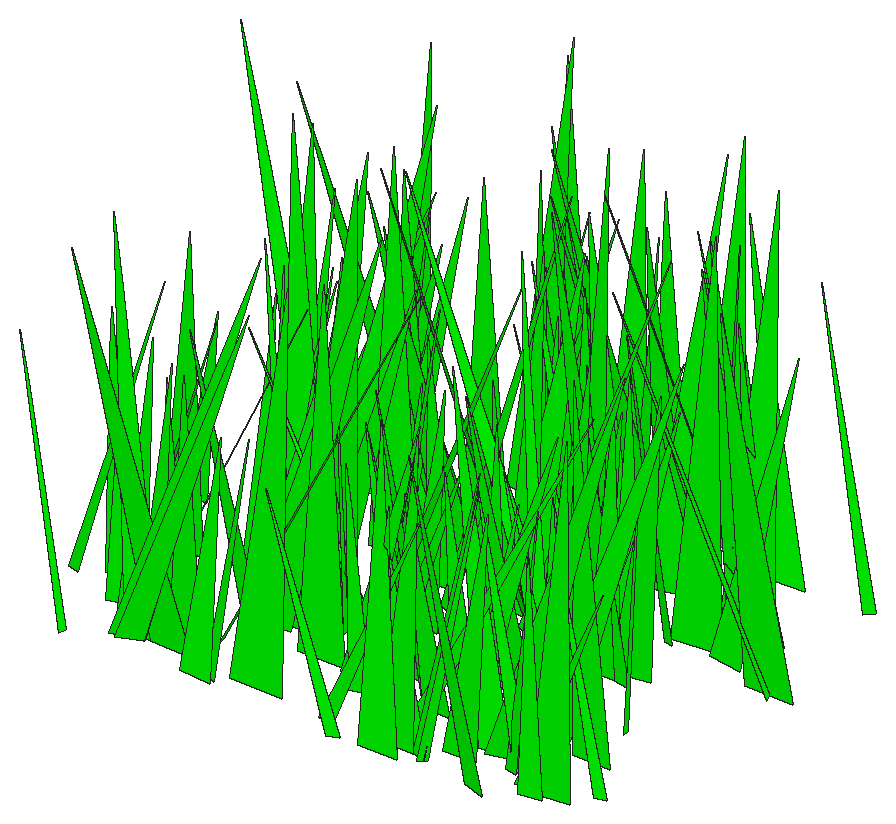
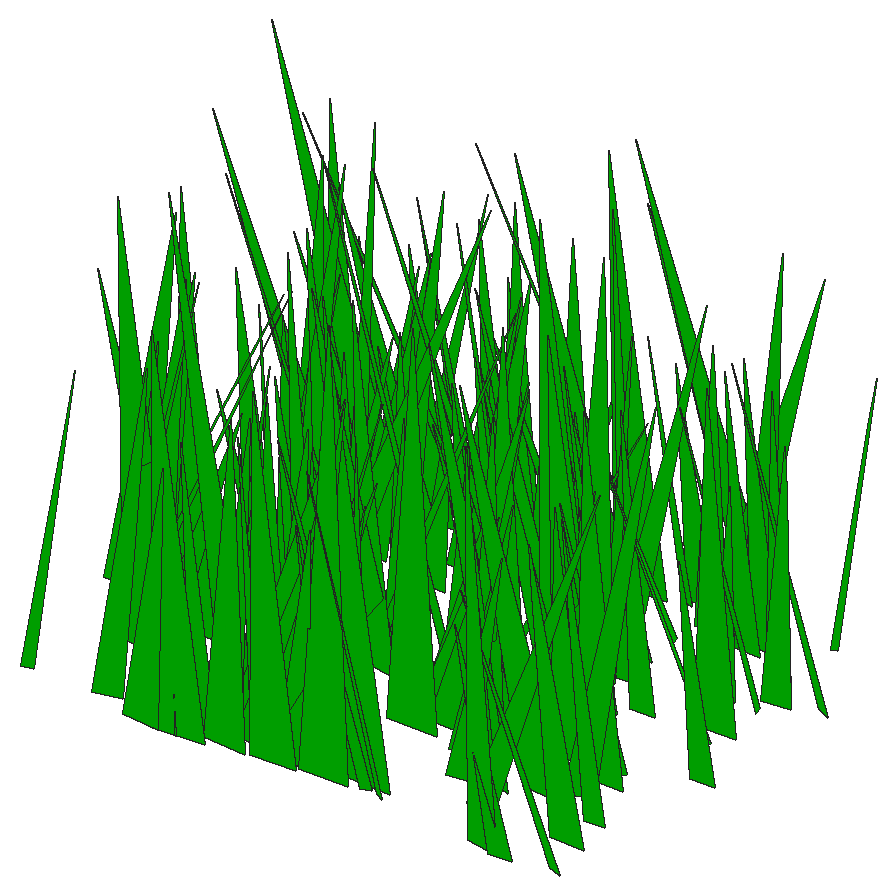
# SketchUp Ruby script. Lengths in inches.
U = 1.inch
M = Sketchup.active_model
def pt(a) = Geom::Point3d.new(a.map { |v| v * U })
def face(e, loops, mat)
  f = e.add_face(loops[0].map { |a| pt(a) })
  loops[1..].each { |l| e.add_face(l.map { |a| pt(a) }).erase! }
  f.material = f.back_material = mat if mat
  f
end
# faces: each face lists its corners as indices into pts; further lists are holes
def faces(e, pts, list, mat = nil) = list.each { |f| face(e, (f[0].is_a?(Array) ? f : [f]).map { |l| l.map { |i| pts[i] } }, mat) }
# xy, xz, yz: faces in a plane at the given z, y or x. An outline is a flat list of corners, or four numbers for a rectangle; further outlines are holes
def ring(l) = l.size == 4 ? [[l[0], l[1]], [l[2], l[1]], [l[2], l[3]], [l[0], l[3]]] : l.each_slice(2).to_a
def flat(e, list, mat, &to3) = list.each { |f| face(e, (f[0].is_a?(Array) ? f : [f]).map { |l| ring(l).map { |u, v| to3.(u, v) } }, mat) }
def xy(e, z, list, mat = nil) = flat(e, list, mat) { |x, y| [x, y, z] }
def xz(e, y, list, mat = nil) = flat(e, list, mat) { |x, z| [x, y, z] }
def yz(e, x, list, mat = nil) = flat(e, list, mat) { |y, z| [x, y, z] }
def lines(e, pts, list) = list.each { |a, b| e.add_line(pt(pts[a]), pt(pts[b])) }
# prism: a flat outline (further loops are holes) pulled along v
def prism(e, loops, v, mat = nil)
  f = face(e, loops, mat); d = Geom::Vector3d.new(v.map { |x| x * U })
  f.pushpull(f.normal.samedirection?(d) ? d.length : -d.length)
end
def box(e, o, s, mat = nil) = prism(e, [[o, [o[0] + s[0], o[1], o[2]], [o[0] + s[0], o[1] + s[1], o[2]], [o[0], o[1] + s[1], o[2]]]], [0, 0, s[2]], mat)
def at(x, y, z, deg = 0) = Geom::Transformation.translation(pt([x, y, z])) * Geom::Transformation.rotation(ORIGIN, Z_AXIS, deg.degrees)
def axes(o, x, y, z) = Geom::Transformation.new([*x, 0, *y, 0, *z, 0, *pt(o).to_a, 1])
def part(name) = M.definitions.add(name)
# library, detail: a bought-in or finely detailed component or shape, given as its bounding box
def library(name, o, s) = part(name).tap { |d| box(d.entities, o, s) }
def detail(e, o, s) = box(e.add_group.entities, o, s)
def put(e, d, t, mat = nil) = e.add_instance(d, t).tap { |i| i.material = mat if mat }
def group(e, t, mat = nil) = e.add_group.tap { |g| g.transformation = t; g.material = mat if mat }.entities
root = M.entities
M.materials.add("[0065_Lime]").color = [0, 255, 0]
c1 = part("fur_instance\#9")
p = [[0.8125,0,1.79],[0.67,-0.02,1.48],[0,-0.11,0],[0,0.11,0]]
faces(c1.entities,p,[[0,1,2,3]])
put(root,c1,axes([28.53,26.51,1.48],[1.94446,-0.52431,0.30164],[3.73909,0.27553,0.10032],[-0.2811,0.03815,3.42098]),"[0065_Lime]")
put(root,c1,axes([30.69,29.18,1.48],[-7.24883,0.59659,1.35662],[-4.26048,-1.0427,0.30299],[1.62965,-0.07228,6.8265]),"[0065_Lime]")
put(root,c1,axes([29.66,21.89,1.48],[2.43602,-0.54167,1.98048],[4.36192,0.38979,0.02249],[-1.32716,0.28686,3.70911]),"[0065_Lime]")
put(root,c1,axes([30.3125,18.52,1.48],[-5.37526,0.04391,1.37175],[-0.43696,-0.7889,-0.28668],[1.65853,-0.06553,4.3703]),"[0065_Lime]")
put(root,c1,axes([29.3,31.42,1.48],[1.7372,0.77211,0.89596],[-5.60051,0.24495,0.11135],[-0.19907,-0.15344,4.68622]),"[0065_Lime]")
put(root,c1,axes([28.375,21.41,1.48],[6.02853,0.28698,0.82516],[-2.03066,0.85892,-0.1937],[-1.03751,-0.01361,5.17381]),"[0065_Lime]")
put(root,c1,axes([29.4,30.12,1.48],[4.78763,-0.38115,1.16224],[2.70623,0.70036,0.32035],[-1.44058,0.04897,4.46442]),"[0065_Lime]")
put(root,c1,axes([28.59,32.84,1.48],[4.66829,0.30685,0.32277],[-2.18537,0.65817,-0.05356],[-0.38739,-0.01522,4.19181]),"[0065_Lime]")
put(root,c1,axes([30.03,24.08,1.48],[0.66516,-0.9095,1.03335],[6.5959,0.0908,-0.13111],[0.03354,0.17988,5.29092]),"[0065_Lime]")
put(root,c1,axes([32.3,31.47,1.48],[-5.59806,-0.65347,0.48872],[4.67301,-0.78835,0.09346],[0.38843,0.0664,5.91905]),"[0065_Lime]")
put(root,c1,axes([30.49,20.73,1.48],[-3.94514,0.41383,2.08396],[-3.38186,-0.61798,-0.12382],[1.94941,-0.23458,4.00264]),"[0065_Lime]")
put(root,c1,axes([30.72,28.24,1.48],[0.06351,1.00668,1.49718],[-7.39594,0.00488,0.09759],[0.10756,-0.25875,5.82675]),"[0065_Lime]")
put(root,c1,axes([31.03,22.45,1.48],[1.96058,-0.48802,0.89851],[3.52754,0.2984,0.33812],[-0.91568,0.10464,3.22638]),"[0065_Lime]")
put(root,c1,axes([29.83,22.45,1.48],[5.47637,0.03064,0.82466],[-0.13545,0.78027,-0.37615],[-1.02812,0.06038,4.44218]),"[0065_Lime]")
put(root,c1,axes([30.23,33.19,1.48],[2.61824,-0.49944,0.0051],[3.55197,0.36771,0.12511],[-0.12755,-0.01211,3.58864]),"[0065_Lime]")
put(root,c1,axes([30.96,33.04,1.48],[5.28712,0.68809,2.30985],[-5.25194,0.79999,-0.03173],[-2.11186,-0.26682,5.86172]),"[0065_Lime]")
put(root,c1,axes([30.54,27.5625,1.48],[4.55578,-0.22354,0.90925],[1.72318,0.64956,-0.3614],[-0.90051,0.11206,3.90849]),"[0065_Lime]")
put(root,c1,axes([32.23,19.62,1.48],[-5.92887,0.69451,1.85297],[-5.05854,-0.87786,0.31647],[2.00728,-0.16093,6.27061]),"[0065_Lime]")
put(root,c1,axes([33.25,19.58,1.48],[-3.84627,-0.95409,0.5057],[6.81766,-0.53944,0.20488],[0.08641,0.09347,6.34419]),"[0065_Lime]")
put(root,c1,axes([29.71,24.71,1.48],[5.7731,0.03624,0.21564],[-0.26747,0.81149,0.16836],[-0.25542,-0.03075,4.69758]),"[0065_Lime]")
put(root,c1,axes([31.66,19.78,1.48],[2.95946,0.67914,1.09682],[-4.91075,0.4372,-0.30431],[-1.03058,-0.13302,4.59976]),"[0065_Lime]")
put(root,c1,axes([32.21,27.77,1.48],[-0.65846,0.74084,0.40123],[-5.28493,-0.09631,0.22017],[0.33079,-0.06396,4.31622]),"[0065_Lime]")
put(root,c1,axes([32.08,20.09,1.48],[3.00252,0.56147,1.53129],[-4.31475,0.44126,0.17608],[-0.94492,-0.23081,4.06171]),"[0065_Lime]")
put(root,c1,axes([31.38,29.75,1.48],[3.30997,1.06959,0.29263],[-7.6179,0.46583,-0.04234],[-0.19124,-0.04344,6.75146]),"[0065_Lime]")
put(root,c1,axes([32.22,24.5,1.48],[4.33729,-0.47684,1.24563],[3.42635,0.64049,0.32223],[-1.45633,0.08675,4.46792]),"[0065_Lime]")
put(root,c1,axes([33.83,30.44,1.48],[-2.98341,0.56809,0.39795],[-4.05646,-0.42208,0.06879],[0.35882,-0.04822,4.08637]),"[0065_Lime]")
put(root,c1,axes([32.56,30.17,1.48],[5.09678,0.33329,1.41012],[-2.41603,0.75303,-0.18614],[-1.67146,-0.07218,4.56892]),"[0065_Lime]")
put(root,c1,axes([33.7,24.95,1.48],[4.55404,-0.88484,3.54342],[7.25802,0.72573,-0.0992],[-2.43922,0.50746,6.32039]),"[0065_Lime]")
put(root,c1,axes([34.61,29.27,1.48],[-3.27427,0.6261,0.62858],[-4.50578,-0.46309,-0.07276],[0.38476,-0.09501,4.49706]),"[0065_Lime]")
put(root,c1,axes([34.05,23.73,1.48],[-6.2833,0.18815,2.07275],[-1.57652,-0.94423,-0.28991],[2.4085,-0.12721,5.21763]),"[0065_Lime]")
put(root,c1,axes([33.74,29.49,1.48],[1.85607,-0.86738,1.7738],[6.48186,0.28817,0.23426],[-0.91846,0.28085,5.23782]),"[0065_Lime]")
put(root,c1,axes([33.59,19.78,1.48],[-1.27012,-0.73073,1.17098],[5.35552,-0.19609,-0.25694],[0.65873,0.18526,4.34675]),"[0065_Lime]")
put(root,c1,axes([32.92,25.06,1.48],[5.95801,-0.23794,1.35455],[1.62666,0.86929,0.38291],[-1.73046,-0.0021,5.02369]),"[0065_Lime]")
put(root,c1,axes([34.58,25.33,1.48],[-3.2959,0.39537,0.88114],[-2.93786,-0.47183,-0.17664],[0.67751,-0.12263,3.52053]),"[0065_Lime]")
put(root,c1,axes([34.32,29.35,1.48],[-2.83799,-0.41183,0.81012],[2.91692,-0.41935,-0.38255],[1.03599,0.05255,3.29636]),"[0065_Lime]")
put(root,c1,axes([32,19.32,1.48],[6.93626,-0.5454,0.40087],[3.86444,0.97705,0.30254],[-0.61157,-0.01192,6.45823]),"[0065_Lime]")
put(root,c1,axes([31.9,19.36,1.48],[7.73818,-0.67451,0.62273],[4.80985,1.09173,0.07932],[-0.70212,0.04502,7.40659]),"[0065_Lime]")
put(root,c1,axes([33.5,23.36,1.48],[1.89489,0.68749,0.51615],[-4.93049,0.26052,0.34847],[0.17399,-0.10477,4.2535]),"[0065_Lime]")
put(root,c1,axes([33.64,25.6,1.48],[1.01521,-1.0318,0.08282],[7.32975,0.14149,-0.38137],[0.45056,0.02317,6.01754]),"[0065_Lime]")
put(root,c1,axes([34.68,27.48,1.48],[-0.23063,1.04261,2.1931],[-7.89444,-0.03172,-0.04394],[0.02632,-0.37892,6.03813]),"[0065_Lime]")
put(root,c1,axes([36.03,20.11,1.48],[3.99965,0.43225,3.3723],[-4.14694,0.70794,0.21354],[-3.07471,-0.39253,4.09875]),"[0065_Lime]")
put(root,c1,axes([36.26,28.41,1.48],[-3.72702,-0.90922,0.02059],[6.46597,-0.52349,-0.21624],[0.24299,-0.01556,6.07]),"[0065_Lime]")
put(root,c1,axes([34.71,18.79,1.48],[-0.08844,0.67947,0.57665],[-4.87322,-0.01979,0.2867],[0.3691,-0.09842,3.92345]),"[0065_Lime]")
put(root,c1,axes([37.39,23.35,1.48],[-5.60505,0.08473,0.07621],[-0.6068,-0.78679,-0.21423],[0.06488,-0.03821,4.58052]),"[0065_Lime]")
put(root,c1,axes([33.75,26.15,1.48],[4.79267,-0.55779,0.71821],[4.03311,0.67653,-0.20055],[-0.52063,0.10603,5.05799]),"[0065_Lime]")
put(root,c1,axes([35.7,24.08,1.48],[-0.55954,-0.6155,0.93138],[4.52001,-0.06669,0.31996],[-0.25857,0.1662,3.57759]),"[0065_Lime]")
put(root,c1,axes([34.34,25,1.48],[2.28445,-1.28329,0.05879],[9.13284,0.32099,-0.01488],[0.00021,0.01048,7.65741]),"[0065_Lime]")
put(root,c1,axes([33.98,28.3,1.48],[5.70355,-0.61239,1.36982],[4.55179,0.81253,-0.36773],[-1.05353,0.19523,5.82706]),"[0065_Lime]")
put(root,c1,axes([36.7,28.6,1.48],[-4.02898,-0.33853,0.43606],[2.44192,-0.56771,0.15975],[0.35826,0.06247,3.81507]),"[0065_Lime]")
put(root,c1,axes([35.05,19,1.48],[4.38399,0.26521,1.15978],[-2.01567,0.63966,0.13987],[-1.2378,-0.10234,3.87989]),"[0065_Lime]")
put(root,c1,axes([35.45,22.61,1.48],[-0.06957,-0.57004,1.65432],[4.524,-0.03113,-0.23356],[0.35594,0.28425,3.29199]),"[0065_Lime]")
put(root,c1,axes([35.97,32.21,1.48],[4.6183,0.51196,2.26448],[-4.10413,0.70913,0.1659],[-2.0446,-0.26704,4.78195]),"[0065_Lime]")
put(root,c1,axes([35.71,20.77,1.48],[-6.79525,0.23703,2.95559],[-2.08303,-1.06784,-0.29908],[3.42187,-0.17934,5.68724]),"[0065_Lime]")
put(root,c1,axes([34.9,32.57,1.48],[5.67197,0.20058,0.98782],[-1.44711,0.81436,-0.04321],[-1.19089,-0.03425,4.75732]),"[0065_Lime]")
put(root,c1,axes([36.37,23.27,1.48],[-4.35434,-0.01055,1.51071],[-0.07069,-0.66331,-0.29006],[1.85742,-0.04998,3.53051]),"[0065_Lime]")
put(root,c1,axes([35.56,32.3,1.48],[4.79175,1.02399,2.56946],[-7.82384,0.6978,0.33523],[-1.36735,-0.4043,7.08626]),"[0065_Lime]")
put(root,c1,axes([36.38,31.375,1.48],[2.96702,0.50866,1.34988],[-3.82227,0.44536,-0.06482],[-1.11723,-0.1728,3.80663]),"[0065_Lime]")
put(root,c1,axes([36.8125,32.4375,1.48],[-0.23189,-0.64567,0.15021],[4.59656,-0.03176,0.12023],[-0.13844,0.02695,3.74041]),"[0065_Lime]")
put(root,c1,axes([34.47,22.27,1.48],[6.51256,-0.9072,0.67586],[6.49078,0.91753,-0.11308],[-0.49174,0.09612,7.45842]),"[0065_Lime]")
put(root,c1,axes([36.83,26.88,1.48],[0.98741,-0.65407,1.11135],[4.81198,0.15688,0.26518],[-0.61465,0.17748,3.86135]),"[0065_Lime]")
put(root,c1,axes([36.76,32.7,1.48],[4.62506,-0.95191,2.59889],[7.18176,0.71342,0.29982],[-2.12642,0.33907,6.66534]),"[0065_Lime]")
put(root,c1,axes([36.625,29.02,1.48],[1.55806,-1.04756,1.22169],[7.58768,0.2286,0.16576],[-0.51046,0.20054,6.19283]),"[0065_Lime]")
put(root,c1,axes([36.79,21.7,1.48],[0.75926,-0.97684,2.03148],[7.3833,0.11116,-0.03475],[-0.22606,0.34955,5.68816]),"[0065_Lime]")
put(root,c1,axes([36.88,31.41,1.48],[0.92233,0.53973,0.86574],[-3.97505,0.13579,-0.03476],[-0.29153,-0.14396,3.21294]),"[0065_Lime]")
put(root,c1,axes([37.8125,32.61,1.48],[4.04253,0.66759,3.26021],[-5.59328,0.68375,-0.10279],[-2.71127,-0.41517,5.07307]),"[0065_Lime]")
put(root,c1,axes([35.43,32.51,1.48],[6.10695,-0.18283,0.75612],[1.2665,0.86783,0.26365],[-0.97622,-0.01785,5.07212]),"[0065_Lime]")
put(root,c1,axes([36.4,19.33,1.48],[2.03662,-1.1052,1.61932],[8.1123,0.28174,-0.30728],[-0.12198,0.28421,6.6015]),"[0065_Lime]")
put(root,c1,axes([38,31.25,1.48],[-4.55192,0.27213,0.98413],[-1.96738,-0.65985,0.09334],[1.15926,-0.05127,4.0227]),"[0065_Lime]")
put(root,c1,axes([36.78,32.58,1.48],[3.88901,0.30023,1.19803],[-2.30479,0.57096,0.15567],[-1.19256,-0.12439,3.60598]),"[0065_Lime]")
put(root,c1,axes([39.76,26.88,1.48],[-7.90485,-0.29025,0.69127],[2.05608,-1.11717,-0.16162],[0.87249,0.00302,6.64383]),"[0065_Lime]")
put(root,c1,axes([34.03,20.81,1.48],[8.91354,0.0453,0.1602],[-0.32063,1.25277,-0.06785],[-0.19983,0.01072,7.25481]),"[0065_Lime]")
put(root,c1,axes([38.07,32.4,1.48],[-2.20873,0.665,0.15589],[-4.71709,-0.31153,0.3104],[0.42686,-0.00164,4.23673]),"[0065_Lime]")
put(root,c1,axes([39.77,32.39,1.48],[-5.30197,-0.49657,0.58348],[3.5638,-0.74892,0.06857],[0.54978,0.06582,5.18242]),"[0065_Lime]")
put(root,c1,axes([37.9,23.63,1.48],[4.21015,-0.36055,1.54275],[2.83885,0.62471,-0.23364],[-1.45665,0.17539,4.00366]),"[0065_Lime]")
put(root,c1,axes([39.9375,32.33,1.48],[-4.98671,-0.78692,0.60293],[5.63015,-0.70369,0.03444],[0.46115,0.08176,6.09936]),"[0065_Lime]")
put(root,c1,axes([37.78,24.78,1.48],[1.57688,-0.67511,0.68009],[4.8758,0.22058,-0.14285],[-0.09145,0.11936,4.11063]),"[0065_Lime]")
put(root,c1,axes([38.74,20.94,1.48],[-2.91327,0.39114,1.36764],[-3.07517,-0.43451,-0.17003],[1.05755,-0.18601,3.27307]),"[0065_Lime]")
put(root,c1,axes([39.71,18.54,1.48],[-4.05107,0.25217,0.51931],[-1.83818,-0.57283,-0.1669],[0.49914,-0.06293,3.60017]),"[0065_Lime]")
put(root,c1,axes([38.35,32.91,1.48],[-0.65086,0.98638,1.60642],[-7.27177,-0.10861,0.28537],[0.54488,-0.27126,5.72725]),"[0065_Lime]")
put(root,c1,axes([38.41,30.25,1.48],[-0.75972,-0.6453,1.26757],[4.8143,-0.12701,-0.25747],[0.58308,0.20788,3.77743]),"[0065_Lime]")
put(root,c1,axes([39.41,22.46,1.48],[-3.19726,-0.46866,0.68811],[3.37743,-0.45847,-0.08013],[0.65757,0.07605,3.75728]),"[0065_Lime]")
put(root,c1,axes([37.52,24.36,1.48],[3.50945,-0.31288,0.0764],[2.21173,0.49199,0.29553],[-0.2737,-0.03608,3.36777]),"[0065_Lime]")
put(root,c1,axes([39.42,31.16,1.48],[-2.30507,0.86836,0.45569],[-6.19787,-0.32624,0.0886],[0.29818,-0.06838,5.36422]),"[0065_Lime]")
put(root,c1,axes([39.23,30.15,1.48],[0.90544,0.74515,0.76373],[-5.35202,0.13937,-0.35847],[-0.59847,-0.11903,4.36116]),"[0065_Lime]")
put(root,c1,axes([38.2,22.65,1.48],[7.05337,-0.04312,1.71477],[0.32901,1.0343,-0.02381],[-2.10478,0.01716,5.74268]),"[0065_Lime]")
put(root,c1,axes([39.28,26.49,1.48],[-2.01259,-0.58607,0.98649],[4.26324,-0.30248,-0.267],[0.83134,0.13237,3.75743]),"[0065_Lime]")
put(root,c1,axes([38.02,21.57,1.48],[4.36753,-0.48476,0.75308],[3.52198,0.61869,-0.1694],[-0.59515,0.10386,4.52402]),"[0065_Lime]")
put(root,c1,axes([40.47,28.75,1.48],[-2.75344,-0.49585,0.34282],[3.55375,-0.38471,0.23901],[0.02603,0.0721,3.6329]),"[0065_Lime]")
put(root,c1,axes([39.08,32.61,1.48],[4.91772,0.34534,1.79891],[-2.77109,0.73434,0.28834],[-1.80335,-0.18666,4.46254]),"[0065_Lime]")
put(root,c1,axes([39.42,27.06,1.48],[3.96284,0.79888,1.60429],[-5.83591,0.59114,-0.32593],[-1.46771,-0.1935,5.6276]),"[0065_Lime]")
put(root,c1,axes([39.96,33.02,1.48],[-0.58145,-0.77648,2.9164],[6.58711,-0.06906,0.25282],[0.00673,0.5057,4.51254]),"[0065_Lime]")
put(root,c1,axes([40.65,21.6,1.48],[-4.88357,-0.41895,1.13883],[3.04797,-0.70816,-0.08162],[1.24862,0.09011,4.65341]),"[0065_Lime]")
put(root,c1,axes([37.29,23.43,1.48],[8.42758,-0.07882,0.79331],[0.59365,1.19128,-0.20633],[-0.95574,0.0449,6.86717]),"[0065_Lime]")
put(root,c1,axes([37.76,25.9375,1.48],[8.66461,0.37962,1.37547],[-2.77369,1.23718,0.11885],[-1.56989,-0.09066,7.38159]),"[0065_Lime]")
put(root,c1,axes([40.3125,32.58,1.48],[-2.66126,-0.79849,0.97958],[5.73938,-0.39013,-0.33953],[0.89454,0.12758,5.09267]),"[0065_Lime]")
put(root,c1,axes([39.74,29.61,1.48],[6.13176,0.71238,2.63894],[-5.5299,0.92372,0.14571],[-2.37644,-0.31137,6.47]),"[0065_Lime]")
put(root,c1,axes([41.35,27.55,1.48],[-5.41512,0.05438,0.8928],[-0.46742,-0.77383,-0.29634],[1.06584,-0.06307,4.40601]),"[0065_Lime]")
put(root,c1,axes([43.11,24.33,1.48],[-8.69176,0.49791,0.45053],[-3.5222,-1.22352,0.35147],[0.67575,0.02697,7.62683]),"[0065_Lime]")
put(root,c1,axes([39.4,26.98,1.48],[2.54907,1.03044,0.27236],[-7.33823,0.35901,-0.07253],[-0.19424,-0.04032,6.31457]),"[0065_Lime]")
put(root,c1,axes([41.47,19.63,1.48],[-3.43856,0.68768,0.42278],[-4.89473,-0.48714,0.21121],[0.51179,-0.03865,4.86054]),"[0065_Lime]")
put(root,c1,axes([39.05,19.0625,1.48],[4.25244,0.35057,0.29883],[-2.51786,0.59587,0.28249],[-0.13985,-0.06827,4.00037]),"[0065_Lime]")
put(root,c1,axes([41.05,22.61,1.48],[0.81393,-0.47745,1.8568],[4.01077,0.15839,0.20153],[-0.81824,0.30147,2.83484]),"[0065_Lime]")
put(root,c1,axes([41.07,21.34,1.48],[-1.22401,-0.61159,0.1991],[4.35713,-0.17276,-0.05922],[0.13644,0.03033,3.67715]),"[0065_Lime]")
put(root,c1,axes([40.86,32.78,1.48],[-2.96023,-0.52485,2.40378],[4.44614,-0.47982,0.11213],[1.70765,0.33946,3.87505]),"[0065_Lime]")
put(root,c1,axes([41.21,18.61,1.48],[-2.63521,0.77249,1.72947],[-5.7719,-0.40453,0.23578],[1.19484,-0.25046,4.95328]),"[0065_Lime]")
put(root,c1,axes([40.88,18.92,1.48],[0.99615,-0.65544,0.99363],[4.82118,0.13814,-0.14457],[-0.07552,0.17313,3.877]),"[0065_Lime]")
put(root,c1,axes([41.28,23.53,1.48],[-0.66332,-0.65636,1.60369],[5.05311,-0.10839,-0.10361],[0.41377,0.27146,3.83616]),"[0065_Lime]")
put(root,c1,axes([41.27,33.37,1.48],[-0.56001,1.12226,1.29652],[-8.1259,-0.092,0.34611],[0.54412,-0.21885,6.50315]),"[0065_Lime]")
put(root,c1,axes([41.39,19.18,1.48],[2.38125,0.77453,1.27062],[-5.67727,0.35091,-0.12798],[-0.76853,-0.19237,4.88235]),"[0065_Lime]")
put(root,c1,axes([41.49,33.33,1.48],[-5.2276,-0.17324,2.23825],[1.38113,-0.8255,-0.00676],[2.68035,0.08748,4.36885]),"[0065_Lime]")
put(root,c1,axes([42.11,27,1.48],[-1.40047,-0.71241,1.32819],[5.29796,-0.21077,-0.0922],[0.54907,0.21667,4.27735]),"[0065_Lime]")
put(root,c1,axes([42.58,33.4,1.48],[-0.57235,0.7592,0.70878],[-5.46165,-0.07141,-0.35483],[-0.34785,-0.12791,4.40511]),"[0065_Lime]")
put(root,c1,axes([41.6,22.54,1.48],[3.62387,-0.28745,0.79713],[2.11208,0.52226,-0.04223],[-0.82711,0.07421,3.38466]),"[0065_Lime]")
put(root,c1,axes([42.5,27.85,1.48],[-1.8154,0.64954,0.87548],[-4.68741,-0.27077,0.30044],[0.74413,-0.12097,4.02836]),"[0065_Lime]")
put(root,c1,axes([41.84,27.14,1.48],[1.89033,-0.64013,0.63137],[4.61949,0.26495,-0.14954],[-0.12539,0.11069,4.0091]),"[0065_Lime]")
put(root,c1,axes([40.12,26.35,1.48],[8.2451,0.34308,0.83176],[-2.46632,1.16639,0.05456],[-0.96127,-0.0499,6.99433]),"[0065_Lime]")
put(root,c1,axes([43.52,22.23,1.48],[-3.39851,-0.74354,0.84072],[5.36541,-0.48328,0.02799],[0.5292,0.12485,5.11534]),"[0065_Lime]")
put(root,c1,axes([43.58,25.79,1.48],[-5.8707,-0.90867,1.71726],[6.58658,-0.85726,-0.30167],[1.70029,0.18341,7.09791]),"[0065_Lime]")
put(root,c1,axes([41.56,30.43,1.48],[7.82172,-0.60216,1.96557],[4.44104,1.13862,-0.00415],[-2.11669,0.1638,7.25459]),"[0065_Lime]")
put(root,c1,axes([42.05,24.82,1.48],[3.02573,-0.69094,0.17166],[4.89697,0.42613,0.36443],[-0.49209,-0.00784,4.68206]),"[0065_Lime]")
put(root,c1,axes([43.72,20.6,1.48],[4.79587,-0.47109,3.43611],[4.3733,0.80454,-0.3425],[-3.15572,0.39902,4.74734]),"[0065_Lime]")
put(root,c1,axes([43.61,28.27,1.48],[-5.2136,-0.21662,1.41487],[1.75554,-0.76042,0.37898],[1.5232,0.13497,4.40605]),"[0065_Lime]")
put(root,c1,axes([43.46,23.04,1.48],[7.63775,-0.26079,3.32699],[2.16719,1.20706,-0.12131],[-3.9341,0.15864,6.39227]),"[0065_Lime]")
put(root,c1,axes([42.15,27.79,1.48],[2.66993,0.57206,0.49713],[-4.11579,0.37313,0.23756],[-0.08843,-0.09437,3.95299]),"[0065_Lime]")
put(root,c1,axes([42.23,19.11,1.48],[5.45343,0.31031,1.15969],[-2.27401,0.78838,0.00645],[-1.31841,-0.07626,4.78578]),"[0065_Lime]")
put(root,c1,axes([46.04,29.64,1.48],[-8.08356,-0.24554,0.43293],[1.73136,-1.13807,-0.23964],[0.58226,-0.02475,6.72288]),"[0065_Lime]")
put(root,c1,axes([44.31,22.44,1.48],[-3.8271,0.39766,0.53725],[-2.834,-0.54468,0.15198],[0.64282,-0.03383,3.86866]),"[0065_Lime]")
put(root,c1,axes([42.5,24.88,1.48],[2.18659,-0.97631,0.15367],[6.95042,0.30729,-0.01467],[-0.0395,0.02608,5.92481]),"[0065_Lime]")
put(root,c1,axes([44.19,32.8125,1.48],[4.53685,-0.47602,3.29928],[4.36992,0.76034,-0.29988],[-2.9718,0.39134,4.59582]),"[0065_Lime]")
put(root,c1,axes([42.44,19.03,1.48],[5.55359,-0.16485,1.1118],[1.16678,0.80351,0.13601],[-1.37229,0.01603,4.61505]),"[0065_Lime]")
put(root,c1,axes([44.54,18.62,1.48],[-5.31383,-0.45166,1.01],[3.19604,-0.7659,-0.35123],[1.28777,0.03714,5.03933]),"[0065_Lime]")
put(root,c1,axes([43.37,25.76,1.48],[1.22229,-0.74992,0.84563],[5.43348,0.17398,-0.02614],[-0.20021,0.14342,4.45339]),"[0065_Lime]")
put(root,c1,axes([43.86,22.91,1.48],[-0.22525,0.61979,0.37128],[-4.43386,-0.03054,-0.07167],[-0.06518,-0.06468,3.59175]),"[0065_Lime]")
put(root,c1,axes([43.09,19.82,1.48],[1.89898,-0.67981,0.70002],[4.91157,0.26656,-0.14126],[-0.15041,0.12154,4.22517]),"[0065_Lime]")
put(root,c1,axes([42.11,21.32,1.48],[5.28356,-0.55535,0.80714],[4.04229,0.74314,-0.37391],[-0.51421,0.13562,5.354]),"[0065_Lime]")
put(root,c1,axes([45.29,28.75,1.48],[-2.74043,-0.55844,0.28852],[3.98987,-0.38322,0.21965],[-0.02186,0.06257,3.92051]),"[0065_Lime]")
put(root,c1,axes([41.13,20.21,1.48],[7.45754,0.40479,0.0606],[-2.88149,1.04717,0.2311],[0.03293,-0.04101,6.4988]),"[0065_Lime]")
put(root,c1,axes([45.08,20.14,1.48],[-4.46812,0.35087,0.91595],[-2.52692,-0.64484,0.12141],[1.05712,-0.05841,4.16167]),"[0065_Lime]")
put(root,c1,axes([45.58,29.44,1.48],[-2.27204,1.0139,1.05092],[-7.33024,-0.31458,-0.31547],[0.01224,-0.18954,6.14517]),"[0065_Lime]")
put(root,c1,axes([46.18,29.91,1.48],[-7.41357,0.07831,1.4047],[-0.53326,-1.06961,0.13593],[1.73448,0.00585,6.04578]),"[0065_Lime]")
put(root,c1,axes([43.98,26.18,1.48],[2.82389,-0.83668,0.0444],[5.94232,0.39652,0.32182],[-0.38084,-0.01691,5.35069]),"[0065_Lime]")
put(root,c1,axes([45.45,29.6,1.48],[-2.16882,-1.00403,0.81091],[7.20916,-0.30722,0.01081],[0.27672,0.13459,6.07387]),"[0065_Lime]")
put(root,c1,axes([44.32,28.61,1.48],[3.54378,-1.06962,1.42599],[7.7458,0.51614,0.23688],[-1.00916,0.20555,6.82569]),"[0065_Lime]")
put(root,c1,axes([47.59,27.65,1.48],[-7.28294,-0.06342,0.26876],[0.43032,-1.02261,-0.37102],[0.35738,-0.06117,5.9238]),"[0065_Lime]")
put(root,c1,axes([45.38,30.14,1.48],[-2.55208,-0.72558,1.50762],[5.42905,-0.37536,0.0271],[0.78984,0.23566,4.68509]),"[0065_Lime]")
put(root,c1,axes([44.71,20.05,1.48],[-4.15341,-0.24048,2.20869],[2.19478,-0.6681,0.29325],[2.34197,0.19962,3.64221]),"[0065_Lime]")
put(root,c1,axes([45.13,29.77,1.48],[1.07811,1.24147,1.22484],[-8.9613,0.15266,0.03391],[-0.14042,-0.21075,7.23973]),"[0065_Lime]")
put(root,c1,axes([46.08,21.83,1.48],[-3.41157,-0.79444,2.50934],[6.33173,-0.50351,0.354],[1.1791,0.40522,5.3595]),"[0065_Lime]")
put(root,c1,axes([45.99,19.28,1.48],[-2.96454,0.4323,1.5573],[-3.37981,-0.45521,-0.02266],[1.30646,-0.19669,3.47512]),"[0065_Lime]")
put(root,c1,axes([45.8125,23.68,1.48],[4.31837,-0.02609,1.38607],[0.10875,0.65188,0.18697],[-1.71064,-0.02442,3.51089]),"[0065_Lime]")
put(root,c1,axes([46.875,32.95,1.48],[-5.75231,0.18509,1.504],[-1.50107,-0.84105,-0.33027],[1.70311,-0.11614,4.78873]),"[0065_Lime]")
put(root,c1,axes([44.26,22.4,1.48],[5.73295,0.88758,0.23161],[-6.31363,0.80651,-0.16577],[-0.3423,-0.01036,6.93661]),"[0065_Lime]")
put(root,c1,axes([44.13,20.56,1.48],[7.11153,-0.8282,0.41633],[5.88368,1.00185,0.28613],[-0.61861,0.00775,7.50761]),"[0065_Lime]")
put(root,c1,axes([45.52,28.36,1.48],[4.02107,0.71079,0.98564],[-5.17581,0.56812,0.24227],[-0.51601,-0.15964,5.25059]),"[0065_Lime]")
put(root,c1,axes([47.57,20.36,1.48],[-4.10308,0.23278,0.80219],[-1.66889,-0.592,0.10857],[0.96527,-0.03404,3.59762]),"[0065_Lime]")
put(root,c1,axes([46.43,19.55,1.48],[3.56139,-0.86142,1.5277],[6.31299,0.52386,0.16084],[-1.11995,0.21367,5.76463]),"[0065_Lime]")
put(root,c1,axes([45.375,19.72,1.48],[4.38098,-0.29278,0.0672],[2.06684,0.61328,0.38249],[-0.27625,-0.05472,3.92746]),"[0065_Lime]")
put(root,c1,axes([47.53,27.75,1.48],[-1.35052,-1.07058,0.63349],[7.65851,-0.1884,0.13367],[-0.02673,0.11178,6.29247]),"[0065_Lime]")
